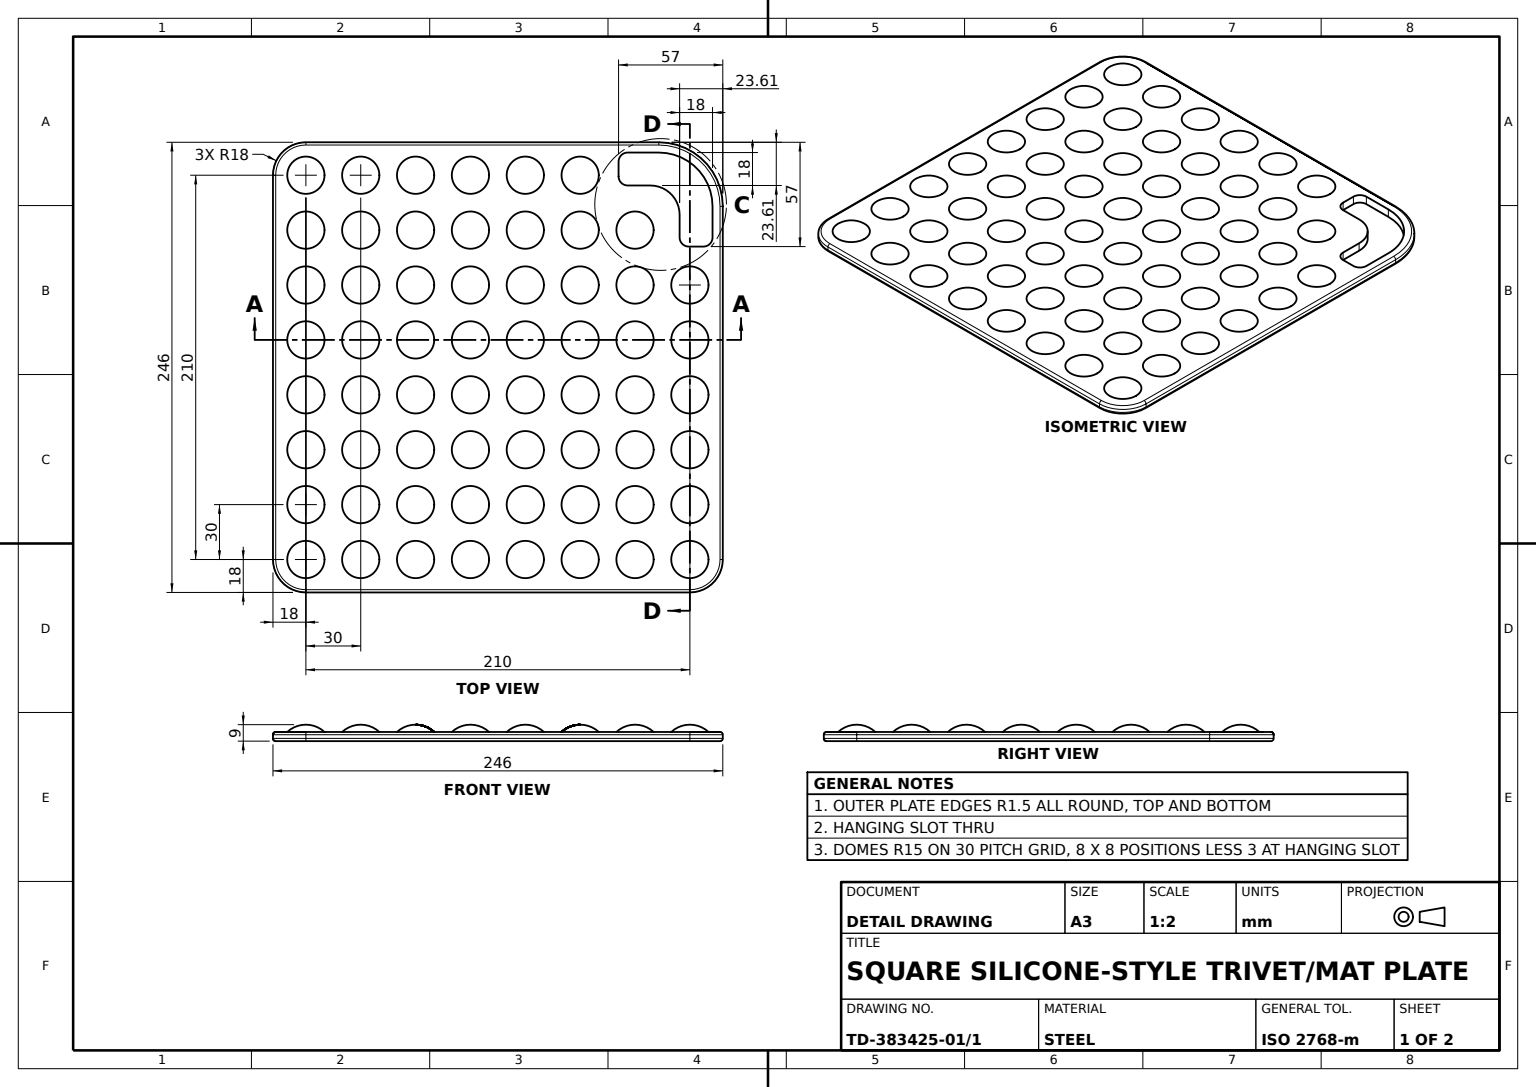
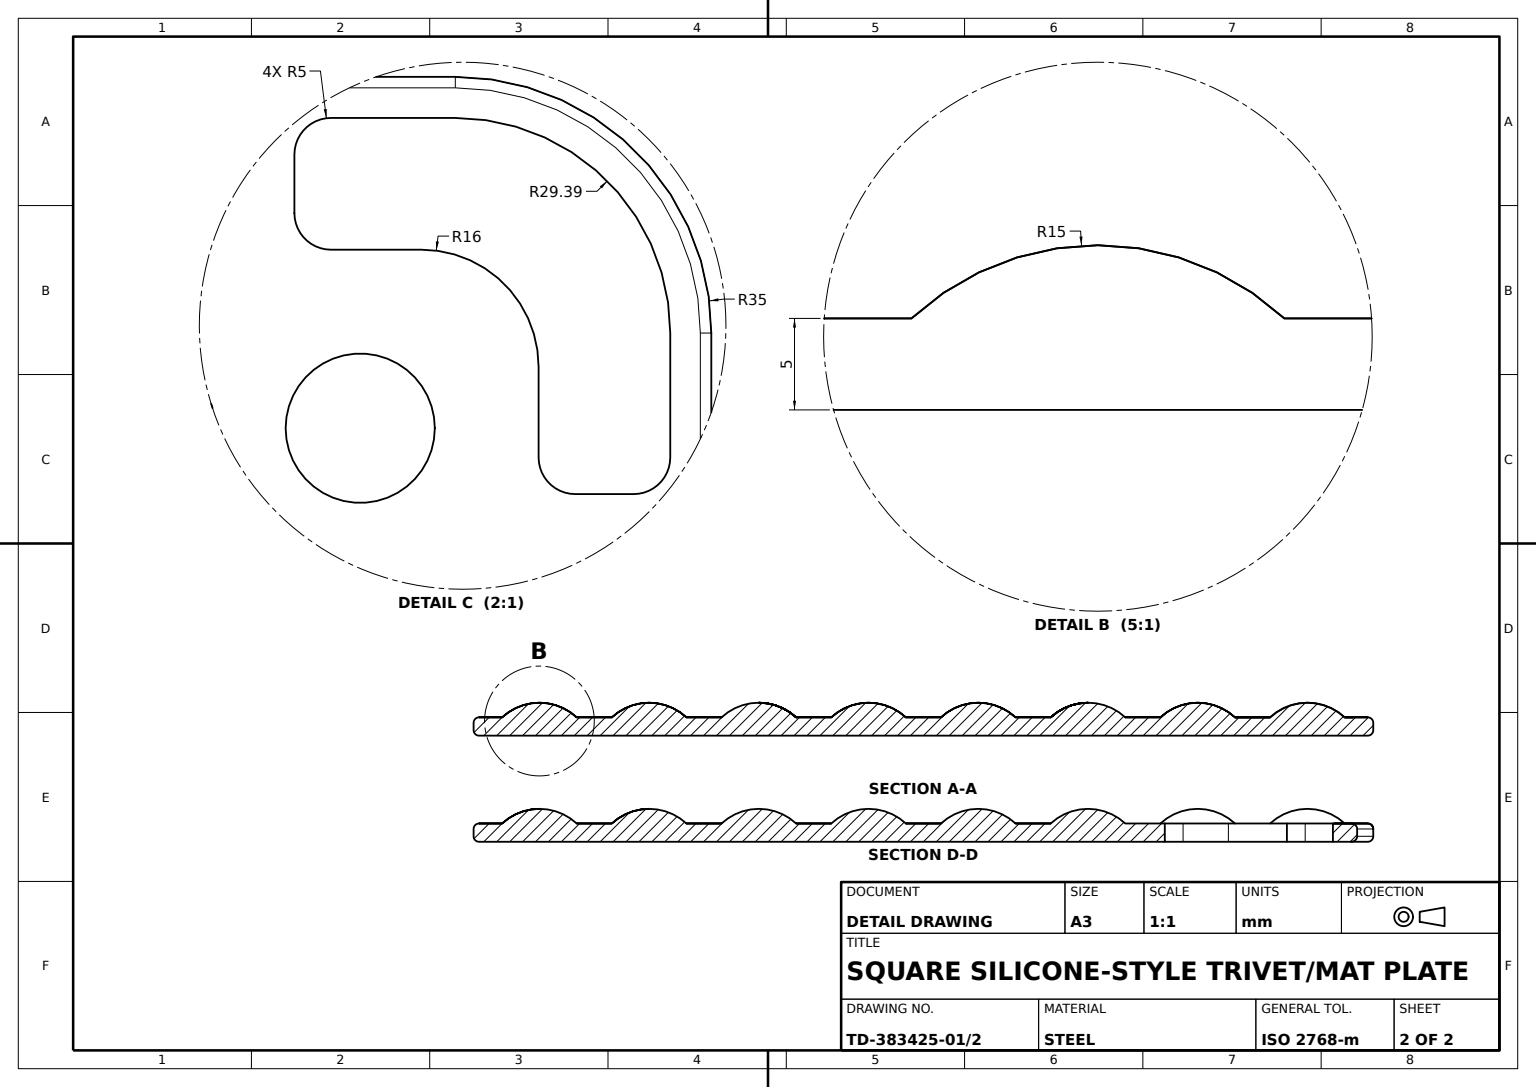
solid
v1 (55.198039,5,-105)
v2 (34.801961,5,-105)
e1 v1 v2 CIRCLE(AX(P(45,5,-105),D(0,1,0),D(0,0,1)),10.198039)
v3 (45,9,-105)
e2 v2 v3 CIRCLE(AX(P(45,-6,-105),D(0,0,-1),D(-1,0,0)),15)
e3 v1 v3 CIRCLE(AX(P(45,-6,-105),D(0,0,1),D(1,0,0)),15)
face SPHERE(AX(P(45,-6,-105),D(0,0,-1),D(1,0,0)),15) [e1 e2 -e3]
v4 (88,5,-121.5)
v5 (-105,5,-121.5)
e4 v4 v5 LINE
v6 (88,3.5,-123)
e5 v6 v4 CIRCLE(AX(P(88,3.5,-121.5),D(1,0,0),D(0,0,-1)),1.5)
v7 (-105,3.5,-123)
e6 v7 v6 LINE
e7 v7 v5 CIRCLE(AX(P(-105,3.5,-121.5),D(1,0,0),D(0,0,-1)),1.5)
face CYL(AX(P(0,3.5,-121.5),D(-1,0,0),D(0,0,1)),1.5) [-e4 -e5 -e6 e7]
v8 (-34.801961,5,-105)
v9 (-55.198039,5,-105)
e8 v8 v9 CIRCLE(AX(P(-45,5,-105),D(0,1,0),D(0,0,1)),10.198039)
v10 (-45,9,-105)
e9 v9 v10 CIRCLE(AX(P(-45,-6,-105),D(0,0,-1),D(-1,0,0)),15)
e10 v8 v10 CIRCLE(AX(P(-45,-6,-105),D(0,0,1),D(1,0,0)),15)
face SPHERE(AX(P(-45,-6,-105),D(0,0,-1),D(1,0,0)),15) [e8 e9 -e10]
v11 (83.387521,0,-99.387521)
v12 (83.387521,5,-99.387521)
e11 v11 v12 LINE
v13 (71,0,-99.387521)
e12 v11 v13 LINE
v14 (71,5,-99.387521)
e13 v13 v14 LINE
e14 v12 v14 LINE
face PLANE(AX(P(71,-7.5,-99.387521),D(0,0,1),D(1,0,0))) rev [-e11 e12 e13 -e14]
v15 (105,1.5,123)
v16 (105,3.5,123)
e15 v15 v16 LINE
v17 (123,1.5,105)
e16 v15 v17 CIRCLE(AX(P(105,1.5,105),D(0,1,0),D(0,0,-1)),18)
v18 (123,3.5,105)
e17 v18 v17 LINE
e18 v18 v16 CIRCLE(AX(P(105,3.5,105),D(0,-1,0),D(0,0,-1)),18)
face CYL(AX(P(105,5,105),D(0,-1,0),D(0,0,-1)),18) [-e15 e16 -e17 e18]
v19 (-64.801961,5,-75)
v20 (-75,9,-75)
e19 v19 v20 CIRCLE(AX(P(-75,-6,-75),D(0,0,1),D(1,0,0)),15)
v21 (-85.198039,5,-75)
e20 v19 v21 CIRCLE(AX(P(-75,5,-75),D(0,1,0),D(0,0,1)),10.198039)
e21 v21 v20 CIRCLE(AX(P(-75,-6,-75),D(0,0,-1),D(-1,0,0)),15)
face SPHERE(AX(P(-75,-6,-75),D(0,0,-1),D(1,0,0)),15) [-e19 e20 e21]
v22 (-55.198039,5,75)
v23 (-45,9,75)
e22 v22 v23 CIRCLE(AX(P(-45,-6,75),D(0,0,-1),D(-1,0,0)),15)
v24 (-34.801961,5,75)
e23 v22 v24 CIRCLE(AX(P(-45,5,75),D(0,1,0),D(0,0,1)),10.198039)
e24 v24 v23 CIRCLE(AX(P(-45,-6,75),D(0,0,1),D(1,0,0)),15)
face SPHERE(AX(P(-45,-6,75),D(0,0,-1),D(1,0,0)),15) [-e22 e23 e24]
v25 (99.387521,0,-71)
v26 (99.387521,5,-71)
e25 v25 v26 LINE
v27 (104.387521,5,-66)
e26 v27 v26 CIRCLE(AX(P(104.387521,5,-71),D(0,-1,0),D(0,0,-1)),5)
v28 (104.387521,0,-66)
e27 v28 v27 LINE
e28 v28 v25 CIRCLE(AX(P(104.387521,0,-71),D(0,-1,0),D(0,0,-1)),5)
face CYL(AX(P(104.387521,-7.5,-71),D(0,1,0),D(0,0,1)),5) rev [e25 -e26 -e27 e28]
v29 (-123,1.5,105)
v30 (-105,1.5,123)
e29 v29 v30 CIRCLE(AX(P(-105,1.5,105),D(0,1,0),D(0,0,-1)),18)
v31 (-121.5,0,105)
e30 v29 v31 CIRCLE(AX(P(-121.5,1.5,105),D(0,0,1),D(1,0,0)),1.5)
v32 (-105,0,121.5)
e31 v32 v31 CIRCLE(AX(P(-105,0,105),D(0,-1,0),D(0,0,-1)),16.5)
e32 v32 v30 CIRCLE(AX(P(-105,1.5,121.5),D(-1,0,0),D(0,0,1)),1.5)
face TORUS(AX(P(-105,1.5,105),D(0,-1,0),D(0,0,-1)),16.5,1.5) [-e29 e30 -e31 e32]
v33 (-34.801961,5,15)
v34 (-45,9,15)
e33 v33 v34 CIRCLE(AX(P(-45,-6,15),D(0,0,1),D(1,0,0)),15)
v35 (-55.198039,5,15)
e34 v33 v35 CIRCLE(AX(P(-45,5,15),D(0,1,0),D(0,0,1)),10.198039)
e35 v35 v34 CIRCLE(AX(P(-45,-6,15),D(0,0,-1),D(-1,0,0)),15)
face SPHERE(AX(P(-45,-6,15),D(0,0,-1),D(1,0,0)),15) [-e33 e34 e35]
v36 (115.198039,5,75)
v37 (94.801961,5,75)
e36 v36 v37 CIRCLE(AX(P(105,5,75),D(0,1,0),D(0,0,1)),10.198039)
v38 (105,9,75)
e37 v37 v38 CIRCLE(AX(P(105,-6,75),D(0,0,-1),D(-1,0,0)),15)
e38 v36 v38 CIRCLE(AX(P(105,-6,75),D(0,0,1),D(1,0,0)),15)
face SPHERE(AX(P(105,-6,75),D(0,0,-1),D(1,0,0)),15) [e36 e37 -e38]
v39 (-115.198039,5,75)
v40 (-105,9,75)
e39 v39 v40 CIRCLE(AX(P(-105,-6,75),D(0,0,-1),D(-1,0,0)),15)
v41 (-94.801961,5,75)
e40 v41 v40 CIRCLE(AX(P(-105,-6,75),D(0,0,1),D(1,0,0)),15)
e41 v41 v39 CIRCLE(AX(P(-105,5,75),D(0,1,0),D(0,0,1)),10.198039)
face SPHERE(AX(P(-105,-6,75),D(0,0,-1),D(1,0,0)),15) [e39 -e40 e41]
v42 (64.801961,5,105)
v43 (75,9,105)
e42 v42 v43 CIRCLE(AX(P(75,-6,105),D(0,0,-1),D(-1,0,0)),15)
v44 (85.198039,5,105)
e43 v42 v44 CIRCLE(AX(P(75,5,105),D(0,1,0),D(0,0,1)),10.198039)
e44 v44 v43 CIRCLE(AX(P(75,-6,105),D(0,0,1),D(1,0,0)),15)
face SPHERE(AX(P(75,-6,105),D(0,0,-1),D(1,0,0)),15) [-e42 e43 e44]
v45 (-85.198039,5,45)
v46 (-64.801961,5,45)
e45 v45 v46 CIRCLE(AX(P(-75,5,45),D(0,1,0),D(0,0,1)),10.198039)
v47 (-75,9,45)
e46 v46 v47 CIRCLE(AX(P(-75,-6,45),D(0,0,1),D(1,0,0)),15)
e47 v45 v47 CIRCLE(AX(P(-75,-6,45),D(0,0,-1),D(-1,0,0)),15)
face SPHERE(AX(P(-75,-6,45),D(0,0,-1),D(1,0,0)),15) [e45 e46 -e47]
v48 (-115.198039,5,-105)
v49 (-94.801961,5,-105)
e48 v48 v49 CIRCLE(AX(P(-105,5,-105),D(0,1,0),D(0,0,1)),10.198039)
v50 (-105,9,-105)
e49 v49 v50 CIRCLE(AX(P(-105,-6,-105),D(0,0,1),D(1,0,0)),15)
e50 v48 v50 CIRCLE(AX(P(-105,-6,-105),D(0,0,-1),D(-1,0,0)),15)
face SPHERE(AX(P(-105,-6,-105),D(0,0,-1),D(1,0,0)),15) [e48 e49 -e50]
e51 v9 v8 CIRCLE(AX(P(-45,5,-105),D(0,1,0),D(0,0,1)),10.198039)
face SPHERE(AX(P(-45,-6,-105),D(0,0,-1),D(1,0,0)),15) [e51 e10 -e9]
v51 (-55.198039,5,-45)
v52 (-34.801961,5,-45)
e52 v51 v52 CIRCLE(AX(P(-45,5,-45),D(0,1,0),D(0,0,1)),10.198039)
v53 (-45,9,-45)
e53 v52 v53 CIRCLE(AX(P(-45,-6,-45),D(0,0,1),D(1,0,0)),15)
e54 v51 v53 CIRCLE(AX(P(-45,-6,-45),D(0,0,-1),D(-1,0,0)),15)
face SPHERE(AX(P(-45,-6,-45),D(0,0,-1),D(1,0,0)),15) [e52 e53 -e54]
v54 (-115.198039,5,45)
v55 (-94.801961,5,45)
e55 v54 v55 CIRCLE(AX(P(-105,5,45),D(0,1,0),D(0,0,1)),10.198039)
v56 (-105,9,45)
e56 v55 v56 CIRCLE(AX(P(-105,-6,45),D(0,0,1),D(1,0,0)),15)
e57 v54 v56 CIRCLE(AX(P(-105,-6,45),D(0,0,-1),D(-1,0,0)),15)
face SPHERE(AX(P(-105,-6,45),D(0,0,-1),D(1,0,0)),15) [e55 e56 -e57]
v57 (85.198039,5,-45)
v58 (75,9,-45)
e58 v57 v58 CIRCLE(AX(P(75,-6,-45),D(0,0,1),D(1,0,0)),15)
v59 (64.801961,5,-45)
e59 v57 v59 CIRCLE(AX(P(75,5,-45),D(0,1,0),D(0,0,1)),10.198039)
e60 v59 v58 CIRCLE(AX(P(75,-6,-45),D(0,0,-1),D(-1,0,0)),15)
face SPHERE(AX(P(75,-6,-45),D(0,0,-1),D(1,0,0)),15) [-e58 e59 e60]
v60 (117.387521,0,-71)
v61 (117.387521,5,-71)
e61 v60 v61 LINE
v62 (112.387521,0,-66)
e62 v60 v62 CIRCLE(AX(P(112.387521,0,-71),D(0,-1,0),D(0,0,-1)),5)
v63 (112.387521,5,-66)
e63 v62 v63 LINE
e64 v61 v63 CIRCLE(AX(P(112.387521,5,-71),D(0,-1,0),D(0,0,-1)),5)
face CYL(AX(P(112.387521,-7.5,-71),D(0,1,0),D(0,0,1)),5) rev [-e61 e62 e63 -e64]
v64 (123,1.5,-88)
e65 v17 v64 LINE
v65 (123,3.5,-88)
e66 v64 v65 LINE
e67 v65 v18 LINE
face PLANE(AX(P(123,5,123),D(-1,0,0),D(0,0,1))) rev [e65 e66 e67 e17]
v66 (-4.801961,5,15)
v67 (-15,9,15)
e68 v66 v67 CIRCLE(AX(P(-15,-6,15),D(0,0,1),D(1,0,0)),15)
v68 (-25.198039,5,15)
e69 v66 v68 CIRCLE(AX(P(-15,5,15),D(0,1,0),D(0,0,1)),10.198039)
e70 v68 v67 CIRCLE(AX(P(-15,-6,15),D(0,0,-1),D(-1,0,0)),15)
face SPHERE(AX(P(-15,-6,15),D(0,0,-1),D(1,0,0)),15) [-e68 e69 e70]
v69 (34.801961,5,-75)
v70 (45,9,-75)
e71 v69 v70 CIRCLE(AX(P(45,-6,-75),D(0,0,-1),D(-1,0,0)),15)
v71 (55.198039,5,-75)
e72 v71 v70 CIRCLE(AX(P(45,-6,-75),D(0,0,1),D(1,0,0)),15)
e73 v71 v69 CIRCLE(AX(P(45,5,-75),D(0,1,0),D(0,0,1)),10.198039)
face SPHERE(AX(P(45,-6,-75),D(0,0,-1),D(1,0,0)),15) [e71 -e72 e73]
v72 (-123,3.5,-105)
e74 v72 v7 CIRCLE(AX(P(-105,3.5,-105),D(0,-1,0),D(0,0,-1)),18)
v73 (-121.5,5,-105)
e75 v73 v72 CIRCLE(AX(P(-121.5,3.5,-105),D(0,0,1),D(1,0,0)),1.5)
e76 v5 v73 CIRCLE(AX(P(-105,5,-105),D(0,1,0),D(0,0,-1)),16.5)
face TORUS(AX(P(-105,3.5,-105),D(0,-1,0),D(0,0,-1)),16.5,1.5) [-e7 -e74 -e75 -e76]
v74 (34.801961,5,15)
v75 (45,9,15)
e77 v74 v75 CIRCLE(AX(P(45,-6,15),D(0,0,-1),D(-1,0,0)),15)
v76 (55.198039,5,15)
e78 v76 v75 CIRCLE(AX(P(45,-6,15),D(0,0,1),D(1,0,0)),15)
e79 v76 v74 CIRCLE(AX(P(45,5,15),D(0,1,0),D(0,0,1)),10.198039)
face SPHERE(AX(P(45,-6,15),D(0,0,-1),D(1,0,0)),15) [e77 -e78 e79]
v77 (-94.801961,5,15)
v78 (-105,9,15)
e80 v77 v78 CIRCLE(AX(P(-105,-6,15),D(0,0,1),D(1,0,0)),15)
v79 (-115.198039,5,15)
e81 v79 v78 CIRCLE(AX(P(-105,-6,15),D(0,0,-1),D(-1,0,0)),15)
e82 v79 v77 CIRCLE(AX(P(-105,5,15),D(0,1,0),D(0,0,1)),10.198039)
face SPHERE(AX(P(-105,-6,15),D(0,0,-1),D(1,0,0)),15) [e80 -e81 e82]
v80 (25.198039,5,-45)
v81 (15,9,-45)
e83 v80 v81 CIRCLE(AX(P(15,-6,-45),D(0,0,1),D(1,0,0)),15)
v82 (4.801961,5,-45)
e84 v80 v82 CIRCLE(AX(P(15,5,-45),D(0,1,0),D(0,0,1)),10.198039)
e85 v82 v81 CIRCLE(AX(P(15,-6,-45),D(0,0,-1),D(-1,0,0)),15)
face SPHERE(AX(P(15,-6,-45),D(0,0,-1),D(1,0,0)),15) [-e83 e84 e85]
e86 v68 v66 CIRCLE(AX(P(-15,5,15),D(0,1,0),D(0,0,1)),10.198039)
face SPHERE(AX(P(-15,-6,15),D(0,0,-1),D(1,0,0)),15) [e86 e68 -e70]
v83 (34.801961,5,-45)
v84 (45,9,-45)
e87 v83 v84 CIRCLE(AX(P(45,-6,-45),D(0,0,-1),D(-1,0,0)),15)
v85 (55.198039,5,-45)
e88 v83 v85 CIRCLE(AX(P(45,5,-45),D(0,1,0),D(0,0,1)),10.198039)
e89 v85 v84 CIRCLE(AX(P(45,-6,-45),D(0,0,1),D(1,0,0)),15)
face SPHERE(AX(P(45,-6,-45),D(0,0,-1),D(1,0,0)),15) [-e87 e88 e89]
e90 v52 v51 CIRCLE(AX(P(-45,5,-45),D(0,1,0),D(0,0,1)),10.198039)
face SPHERE(AX(P(-45,-6,-45),D(0,0,-1),D(1,0,0)),15) [e90 e54 -e53]
v86 (94.801961,5,15)
v87 (105,9,15)
e91 v86 v87 CIRCLE(AX(P(105,-6,15),D(0,0,-1),D(-1,0,0)),15)
v88 (115.198039,5,15)
e92 v86 v88 CIRCLE(AX(P(105,5,15),D(0,1,0),D(0,0,1)),10.198039)
e93 v88 v87 CIRCLE(AX(P(105,-6,15),D(0,0,1),D(1,0,0)),15)
face SPHERE(AX(P(105,-6,15),D(0,0,-1),D(1,0,0)),15) [-e91 e92 e93]
v89 (25.198039,5,105)
v90 (4.801961,5,105)
e94 v89 v90 CIRCLE(AX(P(15,5,105),D(0,1,0),D(0,0,1)),10.198039)
e95 v90 v89 CIRCLE(AX(P(15,5,105),D(0,1,0),D(0,0,1)),10.198039)
v91 (-64.801961,5,-15)
v92 (-85.198039,5,-15)
e96 v91 v92 CIRCLE(AX(P(-75,5,-15),D(0,1,0),D(0,0,1)),10.198039)
e97 v92 v91 CIRCLE(AX(P(-75,5,-15),D(0,1,0),D(0,0,1)),10.198039)
v93 (4.801961,5,45)
v94 (25.198039,5,45)
e98 v93 v94 CIRCLE(AX(P(15,5,45),D(0,1,0),D(0,0,1)),10.198039)
e99 v94 v93 CIRCLE(AX(P(15,5,45),D(0,1,0),D(0,0,1)),10.198039)
e100 v39 v41 CIRCLE(AX(P(-105,5,75),D(0,1,0),D(0,0,1)),10.198039)
v95 (4.801961,5,75)
v96 (25.198039,5,75)
e101 v95 v96 CIRCLE(AX(P(15,5,75),D(0,1,0),D(0,0,1)),10.198039)
e102 v96 v95 CIRCLE(AX(P(15,5,75),D(0,1,0),D(0,0,1)),10.198039)
e103 v82 v80 CIRCLE(AX(P(15,5,-45),D(0,1,0),D(0,0,1)),10.198039)
e104 v24 v22 CIRCLE(AX(P(-45,5,75),D(0,1,0),D(0,0,1)),10.198039)
v97 (-4.801961,5,-105)
v98 (-25.198039,5,-105)
e105 v97 v98 CIRCLE(AX(P(-15,5,-105),D(0,1,0),D(0,0,1)),10.198039)
e106 v98 v97 CIRCLE(AX(P(-15,5,-105),D(0,1,0),D(0,0,1)),10.198039)
v99 (85.198039,5,45)
v100 (64.801961,5,45)
e107 v99 v100 CIRCLE(AX(P(75,5,45),D(0,1,0),D(0,0,1)),10.198039)
e108 v100 v99 CIRCLE(AX(P(75,5,45),D(0,1,0),D(0,0,1)),10.198039)
v101 (64.801961,5,75)
v102 (85.198039,5,75)
e109 v101 v102 CIRCLE(AX(P(75,5,75),D(0,1,0),D(0,0,1)),10.198039)
e110 v102 v101 CIRCLE(AX(P(75,5,75),D(0,1,0),D(0,0,1)),10.198039)
v103 (-94.801961,5,105)
v104 (-115.198039,5,105)
e111 v103 v104 CIRCLE(AX(P(-105,5,105),D(0,1,0),D(0,0,1)),10.198039)
e112 v104 v103 CIRCLE(AX(P(-105,5,105),D(0,1,0),D(0,0,1)),10.198039)
v105 (-55.198039,5,45)
v106 (-34.801961,5,45)
e113 v105 v106 CIRCLE(AX(P(-45,5,45),D(0,1,0),D(0,0,1)),10.198039)
e114 v106 v105 CIRCLE(AX(P(-45,5,45),D(0,1,0),D(0,0,1)),10.198039)
v107 (25.198039,5,15)
v108 (4.801961,5,15)
e115 v107 v108 CIRCLE(AX(P(15,5,15),D(0,1,0),D(0,0,1)),10.198039)
e116 v108 v107 CIRCLE(AX(P(15,5,15),D(0,1,0),D(0,0,1)),10.198039)
v109 (34.801961,5,105)
v110 (55.198039,5,105)
e117 v109 v110 CIRCLE(AX(P(45,5,105),D(0,1,0),D(0,0,1)),10.198039)
e118 v110 v109 CIRCLE(AX(P(45,5,105),D(0,1,0),D(0,0,1)),10.198039)
e119 v21 v19 CIRCLE(AX(P(-75,5,-75),D(0,1,0),D(0,0,1)),10.198039)
e120 v74 v76 CIRCLE(AX(P(45,5,15),D(0,1,0),D(0,0,1)),10.198039)
v111 (-85.198039,5,-45)
v112 (-64.801961,5,-45)
e121 v111 v112 CIRCLE(AX(P(-75,5,-45),D(0,1,0),D(0,0,1)),10.198039)
e122 v112 v111 CIRCLE(AX(P(-75,5,-45),D(0,1,0),D(0,0,1)),10.198039)
v113 (-85.198039,5,-105)
v114 (-64.801961,5,-105)
e123 v113 v114 CIRCLE(AX(P(-75,5,-105),D(0,1,0),D(0,0,1)),10.198039)
e124 v114 v113 CIRCLE(AX(P(-75,5,-105),D(0,1,0),D(0,0,1)),10.198039)
v115 (-85.198039,5,15)
v116 (-64.801961,5,15)
e125 v115 v116 CIRCLE(AX(P(-75,5,15),D(0,1,0),D(0,0,1)),10.198039)
e126 v116 v115 CIRCLE(AX(P(-75,5,15),D(0,1,0),D(0,0,1)),10.198039)
v117 (55.198039,5,45)
v118 (34.801961,5,45)
e127 v117 v118 CIRCLE(AX(P(45,5,45),D(0,1,0),D(0,0,1)),10.198039)
e128 v118 v117 CIRCLE(AX(P(45,5,45),D(0,1,0),D(0,0,1)),10.198039)
e129 v85 v83 CIRCLE(AX(P(45,5,-45),D(0,1,0),D(0,0,1)),10.198039)
e130 v2 v1 CIRCLE(AX(P(45,5,-105),D(0,1,0),D(0,0,1)),10.198039)
e131 v88 v86 CIRCLE(AX(P(105,5,15),D(0,1,0),D(0,0,1)),10.198039)
v119 (-4.801961,5,75)
v120 (-25.198039,5,75)
e132 v119 v120 CIRCLE(AX(P(-15,5,75),D(0,1,0),D(0,0,1)),10.198039)
e133 v120 v119 CIRCLE(AX(P(-15,5,75),D(0,1,0),D(0,0,1)),10.198039)
v121 (115.198039,5,45)
v122 (94.801961,5,45)
e134 v121 v122 CIRCLE(AX(P(105,5,45),D(0,1,0),D(0,0,1)),10.198039)
e135 v122 v121 CIRCLE(AX(P(105,5,45),D(0,1,0),D(0,0,1)),10.198039)
e136 v55 v54 CIRCLE(AX(P(-105,5,45),D(0,1,0),D(0,0,1)),10.198039)
e137 v49 v48 CIRCLE(AX(P(-105,5,-105),D(0,1,0),D(0,0,1)),10.198039)
v123 (25.198039,5,-15)
v124 (4.801961,5,-15)
e138 v123 v124 CIRCLE(AX(P(15,5,-15),D(0,1,0),D(0,0,1)),10.198039)
e139 v124 v123 CIRCLE(AX(P(15,5,-15),D(0,1,0),D(0,0,1)),10.198039)
v125 (-115.198039,5,-75)
v126 (-94.801961,5,-75)
e140 v125 v126 CIRCLE(AX(P(-105,5,-75),D(0,1,0),D(0,0,1)),10.198039)
e141 v126 v125 CIRCLE(AX(P(-105,5,-75),D(0,1,0),D(0,0,1)),10.198039)
v127 (-4.801961,5,-75)
v128 (-25.198039,5,-75)
e142 v127 v128 CIRCLE(AX(P(-15,5,-75),D(0,1,0),D(0,0,1)),10.198039)
e143 v128 v127 CIRCLE(AX(P(-15,5,-75),D(0,1,0),D(0,0,1)),10.198039)
v129 (-55.198039,5,-75)
v130 (-34.801961,5,-75)
e144 v129 v130 CIRCLE(AX(P(-45,5,-75),D(0,1,0),D(0,0,1)),10.198039)
e145 v130 v129 CIRCLE(AX(P(-45,5,-75),D(0,1,0),D(0,0,1)),10.198039)
v131 (-34.801961,5,-15)
v132 (-55.198039,5,-15)
e146 v131 v132 CIRCLE(AX(P(-45,5,-15),D(0,1,0),D(0,0,1)),10.198039)
e147 v132 v131 CIRCLE(AX(P(-45,5,-15),D(0,1,0),D(0,0,1)),10.198039)
e148 v77 v79 CIRCLE(AX(P(-105,5,15),D(0,1,0),D(0,0,1)),10.198039)
v133 (115.198039,5,105)
v134 (94.801961,5,105)
e149 v133 v134 CIRCLE(AX(P(105,5,105),D(0,1,0),D(0,0,1)),10.198039)
e150 v134 v133 CIRCLE(AX(P(105,5,105),D(0,1,0),D(0,0,1)),10.198039)
e151 v44 v42 CIRCLE(AX(P(75,5,105),D(0,1,0),D(0,0,1)),10.198039)
v135 (115.198039,5,-45)
v136 (94.801961,5,-45)
e152 v135 v136 CIRCLE(AX(P(105,5,-45),D(0,1,0),D(0,0,1)),10.198039)
e153 v136 v135 CIRCLE(AX(P(105,5,-45),D(0,1,0),D(0,0,1)),10.198039)
e154 v37 v36 CIRCLE(AX(P(105,5,75),D(0,1,0),D(0,0,1)),10.198039)
v137 (-121.5,5,105)
e155 v73 v137 LINE
v138 (-105,5,121.5)
e156 v137 v138 CIRCLE(AX(P(-105,5,105),D(0,1,0),D(0,0,-1)),16.5)
v139 (105,5,121.5)
e157 v138 v139 LINE
v140 (121.5,5,105)
e158 v139 v140 CIRCLE(AX(P(105,5,105),D(0,1,0),D(0,0,-1)),16.5)
v141 (121.5,5,-88)
e159 v140 v141 LINE
e160 v141 v4 CIRCLE(AX(P(88,5,-88),D(0,1,0),D(0,0,-1)),33.5)
v142 (-25.198039,5,-45)
v143 (-4.801961,5,-45)
e161 v142 v143 CIRCLE(AX(P(-15,5,-45),D(0,1,0),D(0,0,1)),10.198039)
e162 v143 v142 CIRCLE(AX(P(-15,5,-45),D(0,1,0),D(0,0,1)),10.198039)
v144 (-94.801961,5,-45)
v145 (-115.198039,5,-45)
e163 v144 v145 CIRCLE(AX(P(-105,5,-45),D(0,1,0),D(0,0,1)),10.198039)
e164 v145 v144 CIRCLE(AX(P(-105,5,-45),D(0,1,0),D(0,0,1)),10.198039)
v146 (94.801961,5,-15)
v147 (115.198039,5,-15)
e165 v146 v147 CIRCLE(AX(P(105,5,-15),D(0,1,0),D(0,0,1)),10.198039)
e166 v147 v146 CIRCLE(AX(P(105,5,-15),D(0,1,0),D(0,0,1)),10.198039)
v148 (-85.198039,5,75)
v149 (-64.801961,5,75)
e167 v148 v149 CIRCLE(AX(P(-75,5,75),D(0,1,0),D(0,0,1)),10.198039)
e168 v149 v148 CIRCLE(AX(P(-75,5,75),D(0,1,0),D(0,0,1)),10.198039)
v150 (66,5,-104.387521)
v151 (66,5,-112.387521)
e169 v150 v151 LINE
v152 (71,5,-117.387521)
e170 v151 v152 CIRCLE(AX(P(71,5,-112.387521),D(0,-1,0),D(0,0,-1)),5)
v153 (88,5,-117.387521)
e171 v152 v153 LINE
v154 (117.387521,5,-88)
e172 v153 v154 CIRCLE(AX(P(88,5,-88),D(0,-1,0),D(0,0,-1)),29.387521)
e173 v154 v61 LINE
e174 v63 v27 LINE
v155 (99.387521,5,-83.387521)
e175 v26 v155 LINE
e176 v155 v12 CIRCLE(AX(P(83.387521,5,-83.387521),D(0,1,0),D(0,0,-1)),16)
e177 v14 v150 CIRCLE(AX(P(71,5,-104.387521),D(0,-1,0),D(0,0,-1)),5)
v156 (-4.801961,5,45)
v157 (-25.198039,5,45)
e178 v156 v157 CIRCLE(AX(P(-15,5,45),D(0,1,0),D(0,0,1)),10.198039)
e179 v157 v156 CIRCLE(AX(P(-15,5,45),D(0,1,0),D(0,0,1)),10.198039)
e180 v46 v45 CIRCLE(AX(P(-75,5,45),D(0,1,0),D(0,0,1)),10.198039)
v158 (-94.801961,5,-15)
v159 (-115.198039,5,-15)
e181 v158 v159 CIRCLE(AX(P(-105,5,-15),D(0,1,0),D(0,0,1)),10.198039)
e182 v159 v158 CIRCLE(AX(P(-105,5,-15),D(0,1,0),D(0,0,1)),10.198039)
v160 (-4.801961,5,-15)
v161 (-25.198039,5,-15)
e183 v160 v161 CIRCLE(AX(P(-15,5,-15),D(0,1,0),D(0,0,1)),10.198039)
e184 v161 v160 CIRCLE(AX(P(-15,5,-15),D(0,1,0),D(0,0,1)),10.198039)
v162 (-4.801961,5,105)
v163 (-25.198039,5,105)
e185 v162 v163 CIRCLE(AX(P(-15,5,105),D(0,1,0),D(0,0,1)),10.198039)
e186 v163 v162 CIRCLE(AX(P(-15,5,105),D(0,1,0),D(0,0,1)),10.198039)
e187 v59 v57 CIRCLE(AX(P(75,5,-45),D(0,1,0),D(0,0,1)),10.198039)
e188 v69 v71 CIRCLE(AX(P(45,5,-75),D(0,1,0),D(0,0,1)),10.198039)
v164 (25.198039,5,-75)
v165 (4.801961,5,-75)
e189 v164 v165 CIRCLE(AX(P(15,5,-75),D(0,1,0),D(0,0,1)),10.198039)
e190 v165 v164 CIRCLE(AX(P(15,5,-75),D(0,1,0),D(0,0,1)),10.198039)
v166 (-85.198039,5,105)
v167 (-64.801961,5,105)
e191 v166 v167 CIRCLE(AX(P(-75,5,105),D(0,1,0),D(0,0,1)),10.198039)
e192 v167 v166 CIRCLE(AX(P(-75,5,105),D(0,1,0),D(0,0,1)),10.198039)
v168 (34.801961,5,-15)
v169 (55.198039,5,-15)
e193 v168 v169 CIRCLE(AX(P(45,5,-15),D(0,1,0),D(0,0,1)),10.198039)
e194 v169 v168 CIRCLE(AX(P(45,5,-15),D(0,1,0),D(0,0,1)),10.198039)
v170 (4.801961,5,-105)
v171 (25.198039,5,-105)
e195 v170 v171 CIRCLE(AX(P(15,5,-105),D(0,1,0),D(0,0,1)),10.198039)
e196 v171 v170 CIRCLE(AX(P(15,5,-105),D(0,1,0),D(0,0,1)),10.198039)
v172 (85.198039,5,-75)
v173 (64.801961,5,-75)
e197 v172 v173 CIRCLE(AX(P(75,5,-75),D(0,1,0),D(0,0,1)),10.198039)
e198 v173 v172 CIRCLE(AX(P(75,5,-75),D(0,1,0),D(0,0,1)),10.198039)
v174 (55.198039,5,75)
v175 (34.801961,5,75)
e199 v174 v175 CIRCLE(AX(P(45,5,75),D(0,1,0),D(0,0,1)),10.198039)
e200 v175 v174 CIRCLE(AX(P(45,5,75),D(0,1,0),D(0,0,1)),10.198039)
v176 (64.801961,5,15)
v177 (85.198039,5,15)
e201 v176 v177 CIRCLE(AX(P(75,5,15),D(0,1,0),D(0,0,1)),10.198039)
e202 v177 v176 CIRCLE(AX(P(75,5,15),D(0,1,0),D(0,0,1)),10.198039)
e203 v35 v33 CIRCLE(AX(P(-45,5,15),D(0,1,0),D(0,0,1)),10.198039)
v178 (64.801961,5,-15)
v179 (85.198039,5,-15)
e204 v178 v179 CIRCLE(AX(P(75,5,-15),D(0,1,0),D(0,0,1)),10.198039)
e205 v179 v178 CIRCLE(AX(P(75,5,-15),D(0,1,0),D(0,0,1)),10.198039)
v180 (-34.801961,5,105)
v181 (-55.198039,5,105)
e206 v180 v181 CIRCLE(AX(P(-45,5,105),D(0,1,0),D(0,0,1)),10.198039)
e207 v181 v180 CIRCLE(AX(P(-45,5,105),D(0,1,0),D(0,0,1)),10.198039)
face PLANE(AX(P(0,5,0),D(0,-1,0),D(0,0,-1))) rev [-e94 -e95] [-e96 -e97] [-e98 -e99] [-e41 -e100] [-e101 -e102] [-e84 -e103] [-e104 -e23] [-e105 -e106] [-e86 -e69] [-e107 -e108] [-e109 -e110] [-e111 -e112] [-e113 -e114] [-e115 -e116] [-e117 -e118] [-e119 -e20] [-e120 -e79] [-e121 -e122] [-e51 -e8] [-e123 -e124] [-e125 -e126] [-e127 -e128] [-e129 -e88] [-e130 -e1] [-e131 -e92] [-e132 -e133] [-e134 -e135] [-e136 -e55] [-e137 -e48] [-e138 -e139] [-e140 -e141] [-e142 -e143] [-e144 -e145] [-e146 -e147] [-e82 -e148] [-e149 -e150] [-e151 -e43] [-e152 -e153] [-e36 -e154] [e155 e156 e157 e158 e159 e160 e4 e76] [-e161 -e162] [-e163 -e164] [-e165 -e166] [-e167 -e168] [-e90 -e52] [e169 e170 e171 e172 e173 e64 e174 e26 e175 e176 e14 e177] [-e178 -e179] [-e180 -e45] [-e181 -e182] [-e183 -e184] [-e185 -e186] [-e187 -e59] [-e188 -e73] [-e189 -e190] [-e191 -e192] [-e193 -e194] [-e195 -e196] [-e197 -e198] [-e199 -e200] [-e201 -e202] [-e203 -e34] [-e204 -e205] [-e206 -e207]
face SPHERE(AX(P(-75,-6,45),D(0,0,-1),D(1,0,0)),15) [-e46 e180 e47]
face SPHERE(AX(P(45,-6,-105),D(0,0,-1),D(1,0,0)),15) [e130 e3 -e2]
v182 (105,9,45)
e208 v121 v182 CIRCLE(AX(P(105,-6,45),D(0,0,1),D(1,0,0)),15)
e209 v122 v182 CIRCLE(AX(P(105,-6,45),D(0,0,-1),D(-1,0,0)),15)
face SPHERE(AX(P(105,-6,45),D(0,0,-1),D(1,0,0)),15) [e208 -e209 e135]
v183 (-45,9,105)
e210 v180 v183 CIRCLE(AX(P(-45,-6,105),D(0,0,1),D(1,0,0)),15)
e211 v181 v183 CIRCLE(AX(P(-45,-6,105),D(0,0,-1),D(-1,0,0)),15)
face SPHERE(AX(P(-45,-6,105),D(0,0,-1),D(1,0,0)),15) [-e210 e206 e211]
v184 (-123,3.5,105)
e212 v137 v184 CIRCLE(AX(P(-121.5,3.5,105),D(0,0,1),D(1,0,0)),1.5)
v185 (-105,3.5,123)
e213 v185 v184 CIRCLE(AX(P(-105,3.5,105),D(0,-1,0),D(0,0,-1)),18)
e214 v138 v185 CIRCLE(AX(P(-105,3.5,121.5),D(1,0,0),D(0,0,-1)),1.5)
face TORUS(AX(P(-105,3.5,105),D(0,-1,0),D(0,0,-1)),16.5,1.5) [-e156 e212 -e213 -e214]
v186 (-75,9,-105)
e215 v114 v186 CIRCLE(AX(P(-75,-6,-105),D(0,0,1),D(1,0,0)),15)
e216 v113 v186 CIRCLE(AX(P(-75,-6,-105),D(0,0,-1),D(-1,0,0)),15)
face SPHERE(AX(P(-75,-6,-105),D(0,0,-1),D(1,0,0)),15) [e123 e215 -e216]
e217 v65 v141 CIRCLE(AX(P(121.5,3.5,-88),D(0,0,1),D(1,0,0)),1.5)
e218 v6 v65 CIRCLE(AX(P(88,3.5,-88),D(0,-1,0),D(0,0,-1)),35)
face TORUS(AX(P(88,3.5,-88),D(0,-1,0),D(0,0,-1)),33.5,1.5) [e5 -e160 -e217 -e218]
v187 (15,9,-105)
e219 v170 v187 CIRCLE(AX(P(15,-6,-105),D(0,0,-1),D(-1,0,0)),15)
e220 v171 v187 CIRCLE(AX(P(15,-6,-105),D(0,0,1),D(1,0,0)),15)
face SPHERE(AX(P(15,-6,-105),D(0,0,-1),D(1,0,0)),15) [-e219 e195 e220]
v188 (15,9,-15)
e221 v123 v188 CIRCLE(AX(P(15,-6,-15),D(0,0,1),D(1,0,0)),15)
e222 v124 v188 CIRCLE(AX(P(15,-6,-15),D(0,0,-1),D(-1,0,0)),15)
face SPHERE(AX(P(15,-6,-15),D(0,0,-1),D(1,0,0)),15) [e221 -e222 e139]
face SPHERE(AX(P(-45,-6,105),D(0,0,-1),D(1,0,0)),15) [-e211 e207 e210]
v189 (105,0,121.5)
e223 v189 v15 CIRCLE(AX(P(105,1.5,121.5),D(-1,0,0),D(0,0,1)),1.5)
v190 (121.5,0,105)
e224 v190 v189 CIRCLE(AX(P(105,0,105),D(0,-1,0),D(0,0,-1)),16.5)
e225 v190 v17 CIRCLE(AX(P(121.5,1.5,105),D(0,0,1),D(1,0,0)),1.5)
face TORUS(AX(P(105,1.5,105),D(0,-1,0),D(0,0,-1)),16.5,1.5) [-e223 -e224 e225 -e16]
v191 (15,9,45)
e226 v93 v191 CIRCLE(AX(P(15,-6,45),D(0,0,-1),D(-1,0,0)),15)
e227 v94 v191 CIRCLE(AX(P(15,-6,45),D(0,0,1),D(1,0,0)),15)
face SPHERE(AX(P(15,-6,45),D(0,0,-1),D(1,0,0)),15) [-e226 e98 e227]
v192 (105,9,105)
e228 v134 v192 CIRCLE(AX(P(105,-6,105),D(0,0,-1),D(-1,0,0)),15)
e229 v133 v192 CIRCLE(AX(P(105,-6,105),D(0,0,1),D(1,0,0)),15)
face SPHERE(AX(P(105,-6,105),D(0,0,-1),D(1,0,0)),15) [e228 -e229 e149]
v193 (75,9,-75)
e230 v172 v193 CIRCLE(AX(P(75,-6,-75),D(0,0,1),D(1,0,0)),15)
e231 v173 v193 CIRCLE(AX(P(75,-6,-75),D(0,0,-1),D(-1,0,0)),15)
face SPHERE(AX(P(75,-6,-75),D(0,0,-1),D(1,0,0)),15) [e198 e230 -e231]
v194 (-75,9,-45)
e232 v111 v194 CIRCLE(AX(P(-75,-6,-45),D(0,0,-1),D(-1,0,0)),15)
e233 v112 v194 CIRCLE(AX(P(-75,-6,-45),D(0,0,1),D(1,0,0)),15)
face SPHERE(AX(P(-75,-6,-45),D(0,0,-1),D(1,0,0)),15) [e122 e232 -e233]
v195 (-45,9,-15)
e234 v131 v195 CIRCLE(AX(P(-45,-6,-15),D(0,0,1),D(1,0,0)),15)
e235 v132 v195 CIRCLE(AX(P(-45,-6,-15),D(0,0,-1),D(-1,0,0)),15)
face SPHERE(AX(P(-45,-6,-15),D(0,0,-1),D(1,0,0)),15) [e234 -e235 e147]
v196 (-75,9,75)
e236 v149 v196 CIRCLE(AX(P(-75,-6,75),D(0,0,1),D(1,0,0)),15)
e237 v148 v196 CIRCLE(AX(P(-75,-6,75),D(0,0,-1),D(-1,0,0)),15)
face SPHERE(AX(P(-75,-6,75),D(0,0,-1),D(1,0,0)),15) [-e236 e168 e237]
v197 (-75,9,15)
e238 v116 v197 CIRCLE(AX(P(-75,-6,15),D(0,0,1),D(1,0,0)),15)
e239 v115 v197 CIRCLE(AX(P(-75,-6,15),D(0,0,-1),D(-1,0,0)),15)
face SPHERE(AX(P(-75,-6,15),D(0,0,-1),D(1,0,0)),15) [e125 e238 -e239]
e240 v30 v15 LINE
e241 v16 v185 LINE
e242 v185 v30 LINE
face PLANE(AX(P(-123,5,123),D(0,0,-1),D(-1,0,0))) rev [e240 e15 e241 e242]
face SPHERE(AX(P(-75,-6,-105),D(0,0,-1),D(1,0,0)),15) [e124 e216 -e215]
v198 (-15,9,-45)
e243 v143 v198 CIRCLE(AX(P(-15,-6,-45),D(0,0,1),D(1,0,0)),15)
e244 v142 v198 CIRCLE(AX(P(-15,-6,-45),D(0,0,-1),D(-1,0,0)),15)
face SPHERE(AX(P(-15,-6,-45),D(0,0,-1),D(1,0,0)),15) [e161 e243 -e244]
v199 (-75,9,-15)
e245 v91 v199 CIRCLE(AX(P(-75,-6,-15),D(0,0,1),D(1,0,0)),15)
e246 v92 v199 CIRCLE(AX(P(-75,-6,-15),D(0,0,-1),D(-1,0,0)),15)
face SPHERE(AX(P(-75,-6,-15),D(0,0,-1),D(1,0,0)),15) [e245 -e246 e97]
face SPHERE(AX(P(15,-6,-15),D(0,0,-1),D(1,0,0)),15) [e222 -e221 e138]
v200 (-15,9,45)
e247 v156 v200 CIRCLE(AX(P(-15,-6,45),D(0,0,1),D(1,0,0)),15)
e248 v157 v200 CIRCLE(AX(P(-15,-6,45),D(0,0,-1),D(-1,0,0)),15)
face SPHERE(AX(P(-15,-6,45),D(0,0,-1),D(1,0,0)),15) [e179 e247 -e248]
face SPHERE(AX(P(-105,-6,45),D(0,0,-1),D(1,0,0)),15) [-e56 e136 e57]
face SPHERE(AX(P(-75,-6,-45),D(0,0,-1),D(1,0,0)),15) [-e232 e121 e233]
v201 (66,0,-112.387521)
e249 v201 v151 LINE
v202 (71,0,-117.387521)
e250 v201 v202 CIRCLE(AX(P(71,0,-112.387521),D(0,-1,0),D(0,0,-1)),5)
e251 v202 v152 LINE
face CYL(AX(P(71,-7.5,-112.387521),D(0,1,0),D(0,0,1)),5) rev [-e170 -e249 e250 e251]
face SPHERE(AX(P(-45,-6,75),D(0,0,-1),D(1,0,0)),15) [-e24 e104 e22]
v203 (45,9,45)
e252 v117 v203 CIRCLE(AX(P(45,-6,45),D(0,0,1),D(1,0,0)),15)
e253 v118 v203 CIRCLE(AX(P(45,-6,45),D(0,0,-1),D(-1,0,0)),15)
face SPHERE(AX(P(45,-6,45),D(0,0,-1),D(1,0,0)),15) [e128 e252 -e253]
face SPHERE(AX(P(-15,-6,45),D(0,0,-1),D(1,0,0)),15) [e248 -e247 e178]
v204 (-123,1.5,-105)
v205 (-121.5,0,-105)
e254 v204 v205 CIRCLE(AX(P(-121.5,1.5,-105),D(0,0,1),D(1,0,0)),1.5)
e255 v31 v205 LINE
e256 v204 v29 LINE
face CYL(AX(P(-121.5,1.5,123),D(0,0,-1),D(-1,0,0)),1.5) [e254 -e255 -e30 -e256]
v206 (-45,9,45)
e257 v105 v206 CIRCLE(AX(P(-45,-6,45),D(0,0,-1),D(-1,0,0)),15)
e258 v106 v206 CIRCLE(AX(P(-45,-6,45),D(0,0,1),D(1,0,0)),15)
face SPHERE(AX(P(-45,-6,45),D(0,0,-1),D(1,0,0)),15) [e257 -e258 e114]
v207 (117.387521,0,-88)
e259 v207 v154 LINE
e260 v207 v60 LINE
face PLANE(AX(P(117.387521,-7.5,-88),D(1,0,0),D(0,0,-1))) rev [e61 -e173 -e259 e260]
v208 (-15,9,75)
e261 v120 v208 CIRCLE(AX(P(-15,-6,75),D(0,0,-1),D(-1,0,0)),15)
e262 v119 v208 CIRCLE(AX(P(-15,-6,75),D(0,0,1),D(1,0,0)),15)
face SPHERE(AX(P(-15,-6,75),D(0,0,-1),D(1,0,0)),15) [e132 e261 -e262]
v209 (15,9,-75)
e263 v165 v209 CIRCLE(AX(P(15,-6,-75),D(0,0,-1),D(-1,0,0)),15)
e264 v164 v209 CIRCLE(AX(P(15,-6,-75),D(0,0,1),D(1,0,0)),15)
face SPHERE(AX(P(15,-6,-75),D(0,0,-1),D(1,0,0)),15) [-e263 e190 e264]
v210 (88,1.5,-123)
e265 v64 v210 CIRCLE(AX(P(88,1.5,-88),D(0,1,0),D(0,0,-1)),35)
e266 v6 v210 LINE
face CYL(AX(P(88,5,-88),D(0,-1,0),D(0,0,-1)),35) [e218 -e66 e265 -e266]
face SPHERE(AX(P(-45,-6,45),D(0,0,-1),D(1,0,0)),15) [-e257 e113 e258]
v211 (-105,9,105)
e267 v104 v211 CIRCLE(AX(P(-105,-6,105),D(0,0,-1),D(-1,0,0)),15)
e268 v103 v211 CIRCLE(AX(P(-105,-6,105),D(0,0,1),D(1,0,0)),15)
face SPHERE(AX(P(-105,-6,105),D(0,0,-1),D(1,0,0)),15) [e267 -e268 e111]
face SPHERE(AX(P(75,-6,105),D(0,0,-1),D(1,0,0)),15) [e151 e42 -e44]
v212 (66,0,-104.387521)
e269 v212 v201 LINE
e270 v13 v212 CIRCLE(AX(P(71,0,-104.387521),D(0,-1,0),D(0,0,-1)),5)
v213 (99.387521,0,-83.387521)
e271 v213 v11 CIRCLE(AX(P(83.387521,0,-83.387521),D(0,1,0),D(0,0,-1)),16)
e272 v25 v213 LINE
e273 v62 v28 LINE
v214 (88,0,-117.387521)
e274 v214 v207 CIRCLE(AX(P(88,0,-88),D(0,-1,0),D(0,0,-1)),29.387521)
e275 v202 v214 LINE
v215 (-105,0,-121.5)
e276 v205 v215 CIRCLE(AX(P(-105,0,-105),D(0,-1,0),D(0,0,-1)),16.5)
v216 (88,0,-121.5)
e277 v215 v216 LINE
v217 (121.5,0,-88)
e278 v216 v217 CIRCLE(AX(P(88,0,-88),D(0,-1,0),D(0,0,-1)),33.5)
e279 v217 v190 LINE
e280 v189 v32 LINE
face PLANE(AX(P(0,0,0),D(0,-1,0),D(0,0,-1))) [-e250 -e269 -e270 -e12 -e271 -e272 -e28 -e273 -e62 -e260 -e274 -e275] [e31 e255 e276 e277 e278 e279 e224 e280]
v218 (-105,9,-15)
e281 v159 v218 CIRCLE(AX(P(-105,-6,-15),D(0,0,-1),D(-1,0,0)),15)
e282 v158 v218 CIRCLE(AX(P(-105,-6,-15),D(0,0,1),D(1,0,0)),15)
face SPHERE(AX(P(-105,-6,-15),D(0,0,-1),D(1,0,0)),15) [e181 e281 -e282]
face SPHERE(AX(P(105,-6,45),D(0,0,-1),D(1,0,0)),15) [e209 -e208 e134]
face SPHERE(AX(P(45,-6,15),D(0,0,-1),D(1,0,0)),15) [-e77 e120 e78]
face SPHERE(AX(P(15,-6,-105),D(0,0,-1),D(1,0,0)),15) [e196 e219 -e220]
v219 (45,9,-15)
e283 v168 v219 CIRCLE(AX(P(45,-6,-15),D(0,0,-1),D(-1,0,0)),15)
e284 v169 v219 CIRCLE(AX(P(45,-6,-15),D(0,0,1),D(1,0,0)),15)
face SPHERE(AX(P(45,-6,-15),D(0,0,-1),D(1,0,0)),15) [e194 e283 -e284]
v220 (-15,9,-105)
e285 v97 v220 CIRCLE(AX(P(-15,-6,-105),D(0,0,1),D(1,0,0)),15)
e286 v98 v220 CIRCLE(AX(P(-15,-6,-105),D(0,0,-1),D(-1,0,0)),15)
face SPHERE(AX(P(-15,-6,-105),D(0,0,-1),D(1,0,0)),15) [e106 e285 -e286]
e287 v18 v140 CIRCLE(AX(P(121.5,3.5,105),D(0,0,1),D(1,0,0)),1.5)
face CYL(AX(P(121.5,3.5,0),D(0,0,-1),D(-1,0,0)),1.5) [-e287 -e67 e217 -e159]
v221 (-15,9,-15)
e288 v161 v221 CIRCLE(AX(P(-15,-6,-15),D(0,0,-1),D(-1,0,0)),15)
e289 v160 v221 CIRCLE(AX(P(-15,-6,-15),D(0,0,1),D(1,0,0)),15)
face SPHERE(AX(P(-15,-6,-15),D(0,0,-1),D(1,0,0)),15) [e183 e288 -e289]
e290 v213 v155 LINE
face CYL(AX(P(83.387521,-7.5,-83.387521),D(0,1,0),D(0,0,1)),16) [e11 -e176 -e290 e271]
face SPHERE(AX(P(-15,-6,-45),D(0,0,-1),D(1,0,0)),15) [e244 -e243 e162]
face SPHERE(AX(P(-105,-6,75),D(0,0,-1),D(1,0,0)),15) [e40 -e39 e100]
v222 (45,9,105)
e291 v109 v222 CIRCLE(AX(P(45,-6,105),D(0,0,-1),D(-1,0,0)),15)
e292 v110 v222 CIRCLE(AX(P(45,-6,105),D(0,0,1),D(1,0,0)),15)
face SPHERE(AX(P(45,-6,105),D(0,0,-1),D(1,0,0)),15) [e118 e291 -e292]
v223 (15,9,15)
e293 v108 v223 CIRCLE(AX(P(15,-6,15),D(0,0,-1),D(-1,0,0)),15)
e294 v107 v223 CIRCLE(AX(P(15,-6,15),D(0,0,1),D(1,0,0)),15)
face SPHERE(AX(P(15,-6,15),D(0,0,-1),D(1,0,0)),15) [-e293 e116 e294]
face SPHERE(AX(P(45,-6,45),D(0,0,-1),D(1,0,0)),15) [e127 e253 -e252]
v224 (-15,9,105)
e295 v162 v224 CIRCLE(AX(P(-15,-6,105),D(0,0,1),D(1,0,0)),15)
e296 v163 v224 CIRCLE(AX(P(-15,-6,105),D(0,0,-1),D(-1,0,0)),15)
face SPHERE(AX(P(-15,-6,105),D(0,0,-1),D(1,0,0)),15) [e186 e295 -e296]
v225 (-105,1.5,-123)
e297 v225 v204 CIRCLE(AX(P(-105,1.5,-105),D(0,1,0),D(0,0,-1)),18)
e298 v225 v215 CIRCLE(AX(P(-105,1.5,-121.5),D(-1,0,0),D(0,0,1)),1.5)
face TORUS(AX(P(-105,1.5,-105),D(0,-1,0),D(0,0,-1)),16.5,1.5) [-e297 e298 -e276 -e254]
face SPHERE(AX(P(-75,-6,-75),D(0,0,-1),D(1,0,0)),15) [e119 e19 -e21]
e299 v210 v225 LINE
e300 v210 v216 CIRCLE(AX(P(88,1.5,-121.5),D(-1,0,0),D(0,0,1)),1.5)
face CYL(AX(P(-123,1.5,-121.5),D(1,0,0),D(0,0,-1)),1.5) [-e299 e300 -e277 -e298]
face SPHERE(AX(P(15,-6,15),D(0,0,-1),D(1,0,0)),15) [e115 e293 -e294]
face SPHERE(AX(P(-105,-6,15),D(0,0,-1),D(1,0,0)),15) [e81 -e80 e148]
face SPHERE(AX(P(-15,-6,-105),D(0,0,-1),D(1,0,0)),15) [e286 -e285 e105]
e301 v184 v72 LINE
face CYL(AX(P(-121.5,3.5,0),D(0,0,1),D(1,0,0)),1.5) [-e155 e75 -e301 -e212]
v226 (15,9,75)
e302 v95 v226 CIRCLE(AX(P(15,-6,75),D(0,0,-1),D(-1,0,0)),15)
e303 v96 v226 CIRCLE(AX(P(15,-6,75),D(0,0,1),D(1,0,0)),15)
face SPHERE(AX(P(15,-6,75),D(0,0,-1),D(1,0,0)),15) [e102 e302 -e303]
face PLANE(AX(P(112.387521,-7.5,-66),D(0,0,1),D(1,0,0))) rev [-e63 e273 e27 -e174]
v227 (-105,9,-45)
e304 v145 v227 CIRCLE(AX(P(-105,-6,-45),D(0,0,-1),D(-1,0,0)),15)
e305 v144 v227 CIRCLE(AX(P(-105,-6,-45),D(0,0,1),D(1,0,0)),15)
face SPHERE(AX(P(-105,-6,-45),D(0,0,-1),D(1,0,0)),15) [e304 -e305 e163]
e306 v225 v7 LINE
face PLANE(AX(P(-123,5,-123),D(0,0,1),D(1,0,0))) rev [e306 e6 e266 e299]
face SPHERE(AX(P(-45,-6,-15),D(0,0,-1),D(1,0,0)),15) [-e234 e146 e235]
e307 v139 v16 CIRCLE(AX(P(105,3.5,121.5),D(1,0,0),D(0,0,-1)),1.5)
face CYL(AX(P(0,3.5,121.5),D(1,0,0),D(0,0,-1)),1.5) [-e307 -e157 e214 -e241]
v228 (75,9,45)
e308 v99 v228 CIRCLE(AX(P(75,-6,45),D(0,0,1),D(1,0,0)),15)
e309 v100 v228 CIRCLE(AX(P(75,-6,45),D(0,0,-1),D(-1,0,0)),15)
face SPHERE(AX(P(75,-6,45),D(0,0,-1),D(1,0,0)),15) [e308 -e309 e108]
e310 v217 v64 CIRCLE(AX(P(121.5,1.5,-88),D(0,0,1),D(1,0,0)),1.5)
face TORUS(AX(P(88,1.5,-88),D(0,-1,0),D(0,0,-1)),33.5,1.5) [-e300 -e265 -e310 -e278]
face CYL(AX(P(-123,1.5,121.5),D(-1,0,0),D(0,0,1)),1.5) [-e240 -e32 -e280 e223]
face SPHERE(AX(P(-105,-6,-45),D(0,0,-1),D(1,0,0)),15) [e305 -e304 e164]
v229 (-105,9,-75)
e311 v126 v229 CIRCLE(AX(P(-105,-6,-75),D(0,0,1),D(1,0,0)),15)
e312 v125 v229 CIRCLE(AX(P(-105,-6,-75),D(0,0,-1),D(-1,0,0)),15)
face SPHERE(AX(P(-105,-6,-75),D(0,0,-1),D(1,0,0)),15) [e140 e311 -e312]
face SPHERE(AX(P(105,-6,15),D(0,0,-1),D(1,0,0)),15) [e91 -e93 e131]
v230 (75,9,-15)
e313 v179 v230 CIRCLE(AX(P(75,-6,-15),D(0,0,1),D(1,0,0)),15)
e314 v178 v230 CIRCLE(AX(P(75,-6,-15),D(0,0,-1),D(-1,0,0)),15)
face SPHERE(AX(P(75,-6,-15),D(0,0,-1),D(1,0,0)),15) [e313 -e314 e204]
v231 (-45,9,-75)
e315 v130 v231 CIRCLE(AX(P(-45,-6,-75),D(0,0,1),D(1,0,0)),15)
e316 v129 v231 CIRCLE(AX(P(-45,-6,-75),D(0,0,-1),D(-1,0,0)),15)
face SPHERE(AX(P(-45,-6,-75),D(0,0,-1),D(1,0,0)),15) [-e315 e145 e316]
face SPHERE(AX(P(45,-6,-15),D(0,0,-1),D(1,0,0)),15) [e284 -e283 e193]
face SPHERE(AX(P(45,-6,-75),D(0,0,-1),D(1,0,0)),15) [-e71 e188 e72]
face SPHERE(AX(P(-105,-6,-15),D(0,0,-1),D(1,0,0)),15) [-e281 e182 e282]
face CYL(AX(P(121.5,1.5,123),D(0,0,1),D(1,0,0)),1.5) [e310 -e65 -e225 -e279]
face SPHERE(AX(P(75,-6,-45),D(0,0,-1),D(1,0,0)),15) [e187 e58 -e60]
v232 (-15,9,-75)
e317 v127 v232 CIRCLE(AX(P(-15,-6,-75),D(0,0,1),D(1,0,0)),15)
e318 v128 v232 CIRCLE(AX(P(-15,-6,-75),D(0,0,-1),D(-1,0,0)),15)
face SPHERE(AX(P(-15,-6,-75),D(0,0,-1),D(1,0,0)),15) [e143 e317 -e318]
face SPHERE(AX(P(-75,-6,-15),D(0,0,-1),D(1,0,0)),15) [e96 e246 -e245]
face TORUS(AX(P(105,3.5,105),D(0,-1,0),D(0,0,-1)),16.5,1.5) [e307 -e18 e287 -e158]
e319 v29 v184 LINE
e320 v72 v204 LINE
face PLANE(AX(P(-123,5,123),D(1,0,0),D(0,0,-1))) rev [e319 e301 e320 e256]
face SPHERE(AX(P(105,-6,105),D(0,0,-1),D(1,0,0)),15) [e229 -e228 e150]
face SPHERE(AX(P(-75,-6,75),D(0,0,-1),D(1,0,0)),15) [e167 e236 -e237]
face SPHERE(AX(P(45,-6,105),D(0,0,-1),D(1,0,0)),15) [e292 -e291 e117]
v233 (45,9,75)
e321 v174 v233 CIRCLE(AX(P(45,-6,75),D(0,0,1),D(1,0,0)),15)
e322 v175 v233 CIRCLE(AX(P(45,-6,75),D(0,0,-1),D(-1,0,0)),15)
face SPHERE(AX(P(45,-6,75),D(0,0,-1),D(1,0,0)),15) [e321 -e322 e200]
v234 (-75,9,105)
e323 v167 v234 CIRCLE(AX(P(-75,-6,105),D(0,0,1),D(1,0,0)),15)
e324 v166 v234 CIRCLE(AX(P(-75,-6,105),D(0,0,-1),D(-1,0,0)),15)
face SPHERE(AX(P(-75,-6,105),D(0,0,-1),D(1,0,0)),15) [-e323 e192 e324]
face SPHERE(AX(P(15,-6,45),D(0,0,-1),D(1,0,0)),15) [e99 e226 -e227]
face SPHERE(AX(P(-15,-6,105),D(0,0,-1),D(1,0,0)),15) [-e295 e185 e296]
v235 (105,9,-45)
e325 v135 v235 CIRCLE(AX(P(105,-6,-45),D(0,0,1),D(1,0,0)),15)
e326 v136 v235 CIRCLE(AX(P(105,-6,-45),D(0,0,-1),D(-1,0,0)),15)
face SPHERE(AX(P(105,-6,-45),D(0,0,-1),D(1,0,0)),15) [e325 -e326 e153]
v236 (75,9,15)
e327 v176 v236 CIRCLE(AX(P(75,-6,15),D(0,0,-1),D(-1,0,0)),15)
e328 v177 v236 CIRCLE(AX(P(75,-6,15),D(0,0,1),D(1,0,0)),15)
face SPHERE(AX(P(75,-6,15),D(0,0,-1),D(1,0,0)),15) [e202 e327 -e328]
face SPHERE(AX(P(45,-6,-45),D(0,0,-1),D(1,0,0)),15) [e87 -e89 e129]
v237 (105,9,-15)
e329 v146 v237 CIRCLE(AX(P(105,-6,-15),D(0,0,-1),D(-1,0,0)),15)
e330 v147 v237 CIRCLE(AX(P(105,-6,-15),D(0,0,1),D(1,0,0)),15)
face SPHERE(AX(P(105,-6,-15),D(0,0,-1),D(1,0,0)),15) [e329 -e330 e166]
face SPHERE(AX(P(75,-6,15),D(0,0,-1),D(1,0,0)),15) [-e327 e201 e328]
v238 (75,9,75)
e331 v101 v238 CIRCLE(AX(P(75,-6,75),D(0,0,-1),D(-1,0,0)),15)
e332 v102 v238 CIRCLE(AX(P(75,-6,75),D(0,0,1),D(1,0,0)),15)
face SPHERE(AX(P(75,-6,75),D(0,0,-1),D(1,0,0)),15) [-e331 e109 e332]
face SPHERE(AX(P(45,-6,75),D(0,0,-1),D(1,0,0)),15) [e322 -e321 e199]
v239 (15,9,105)
e333 v89 v239 CIRCLE(AX(P(15,-6,105),D(0,0,1),D(1,0,0)),15)
e334 v90 v239 CIRCLE(AX(P(15,-6,105),D(0,0,-1),D(-1,0,0)),15)
face SPHERE(AX(P(15,-6,105),D(0,0,-1),D(1,0,0)),15) [e333 -e334 e95]
face SPHERE(AX(P(75,-6,-75),D(0,0,-1),D(1,0,0)),15) [e197 e231 -e230]
face SPHERE(AX(P(15,-6,-75),D(0,0,-1),D(1,0,0)),15) [e189 e263 -e264]
face SPHERE(AX(P(75,-6,45),D(0,0,-1),D(1,0,0)),15) [e107 e309 -e308]
e335 v212 v150 LINE
face CYL(AX(P(71,-7.5,-104.387521),D(0,1,0),D(0,0,1)),5) rev [-e177 -e13 e270 e335]
face SPHERE(AX(P(15,-6,-45),D(0,0,-1),D(1,0,0)),15) [e83 -e85 e103]
face SPHERE(AX(P(15,-6,75),D(0,0,-1),D(1,0,0)),15) [e101 e303 -e302]
face SPHERE(AX(P(105,-6,-45),D(0,0,-1),D(1,0,0)),15) [-e325 e152 e326]
e336 v214 v153 LINE
face CYL(AX(P(88,-7.5,-88),D(0,1,0),D(0,0,1)),29.387521) rev [e259 -e172 -e336 e274]
face SPHERE(AX(P(-75,-6,105),D(0,0,-1),D(1,0,0)),15) [e191 e323 -e324]
face SPHERE(AX(P(-15,-6,-15),D(0,0,-1),D(1,0,0)),15) [e184 e289 -e288]
face SPHERE(AX(P(15,-6,105),D(0,0,-1),D(1,0,0)),15) [e94 e334 -e333]
face SPHERE(AX(P(-105,-6,105),D(0,0,-1),D(1,0,0)),15) [e112 e268 -e267]
face SPHERE(AX(P(-105,-6,-105),D(0,0,-1),D(1,0,0)),15) [-e49 e137 e50]
face SPHERE(AX(P(-15,-6,-75),D(0,0,-1),D(1,0,0)),15) [e142 e318 -e317]
face SPHERE(AX(P(-45,-6,-75),D(0,0,-1),D(1,0,0)),15) [e315 -e316 e144]
face CYL(AX(P(-105,5,-105),D(0,-1,0),D(0,0,-1)),18) [e74 -e306 e297 -e320]
face SPHERE(AX(P(-75,-6,15),D(0,0,-1),D(1,0,0)),15) [-e238 e126 e239]
face SPHERE(AX(P(105,-6,75),D(0,0,-1),D(1,0,0)),15) [-e37 e154 e38]
face SPHERE(AX(P(-15,-6,75),D(0,0,-1),D(1,0,0)),15) [e133 e262 -e261]
face SPHERE(AX(P(75,-6,-15),D(0,0,-1),D(1,0,0)),15) [e314 -e313 e205]
face SPHERE(AX(P(-105,-6,-75),D(0,0,-1),D(1,0,0)),15) [e141 e312 -e311]
face PLANE(AX(P(99.387521,-7.5,-71),D(-1,0,0),D(0,0,1))) rev [e272 e290 -e175 -e25]
face CYL(AX(P(-105,5,105),D(0,-1,0),D(0,0,-1)),18) [-e242 e213 -e319 e29]
face SPHERE(AX(P(105,-6,-15),D(0,0,-1),D(1,0,0)),15) [e330 -e329 e165]
face PLANE(AX(P(66,-7.5,-112.387521),D(-1,0,0),D(0,0,1))) rev [-e169 -e335 e269 e249]
face SPHERE(AX(P(75,-6,75),D(0,0,-1),D(1,0,0)),15) [e331 -e332 e110]
face PLANE(AX(P(88,-7.5,-117.387521),D(0,0,-1),D(-1,0,0))) rev [-e251 e275 e336 -e171]
face SPHERE(AX(P(-45,-6,15),D(0,0,-1),D(1,0,0)),15) [e203 e33 -e35]
